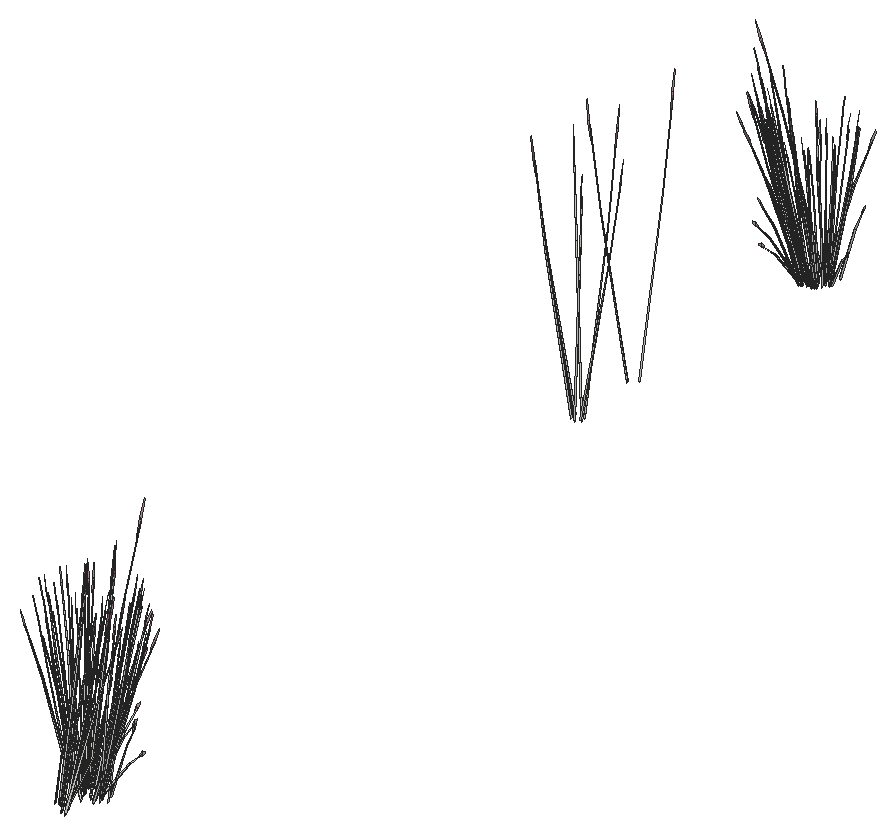
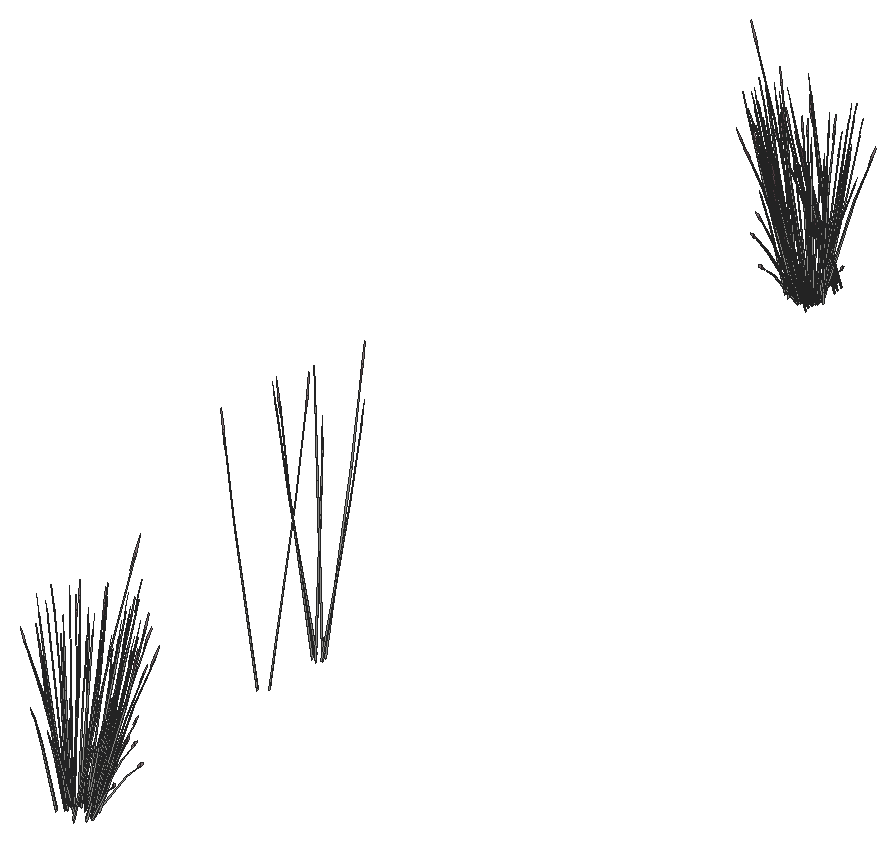
# SketchUp Ruby script. Lengths in inches.
U = 1.inch
M = Sketchup.active_model
def pt(a) = Geom::Point3d.new(a.map { |v| v * U })
def face(e, loops, mat)
  f = e.add_face(loops[0].map { |a| pt(a) })
  loops[1..].each { |l| e.add_face(l.map { |a| pt(a) }).erase! }
  f.material = f.back_material = mat if mat
  f
end
# faces: each face lists its corners as indices into pts; further lists are holes
def faces(e, pts, list, mat = nil) = list.each { |f| face(e, (f[0].is_a?(Array) ? f : [f]).map { |l| l.map { |i| pts[i] } }, mat) }
# xy, xz, yz: faces in a plane at the given z, y or x. An outline is a flat list of corners, or four numbers for a rectangle; further outlines are holes
def ring(l) = l.size == 4 ? [[l[0], l[1]], [l[2], l[1]], [l[2], l[3]], [l[0], l[3]]] : l.each_slice(2).to_a
def flat(e, list, mat, &to3) = list.each { |f| face(e, (f[0].is_a?(Array) ? f : [f]).map { |l| ring(l).map { |u, v| to3.(u, v) } }, mat) }
def xy(e, z, list, mat = nil) = flat(e, list, mat) { |x, y| [x, y, z] }
def xz(e, y, list, mat = nil) = flat(e, list, mat) { |x, z| [x, y, z] }
def yz(e, x, list, mat = nil) = flat(e, list, mat) { |y, z| [x, y, z] }
def lines(e, pts, list) = list.each { |a, b| e.add_line(pt(pts[a]), pt(pts[b])) }
# prism: a flat outline (further loops are holes) pulled along v
def prism(e, loops, v, mat = nil)
  f = face(e, loops, mat); d = Geom::Vector3d.new(v.map { |x| x * U })
  f.pushpull(f.normal.samedirection?(d) ? d.length : -d.length)
end
def box(e, o, s, mat = nil) = prism(e, [[o, [o[0] + s[0], o[1], o[2]], [o[0] + s[0], o[1] + s[1], o[2]], [o[0], o[1] + s[1], o[2]]]], [0, 0, s[2]], mat)
def at(x, y, z, deg = 0) = Geom::Transformation.translation(pt([x, y, z])) * Geom::Transformation.rotation(ORIGIN, Z_AXIS, deg.degrees)
def axes(o, x, y, z) = Geom::Transformation.new([*x, 0, *y, 0, *z, 0, *pt(o).to_a, 1])
def part(name) = M.definitions.add(name)
# library, detail: a bought-in or finely detailed component or shape, given as its bounding box
def library(name, o, s) = part(name).tap { |d| box(d.entities, o, s) }
def detail(e, o, s) = box(e.add_group.entities, o, s)
def put(e, d, t, mat = nil) = e.add_instance(d, t).tap { |i| i.material = mat if mat }
def group(e, t, mat = nil) = e.add_group.tap { |g| g.transformation = t; g.material = mat if mat }.entities
root = M.entities
M.materials.add("LightPink_Translucent").color = [144, 107, 117]
M.materials["LightPink_Translucent"].alpha = 0.75
c1 = part("blade")
p = [[2.15,0.21,22],[0,0.17,0],[0.09,0.45,0],[2.18,0.31,22],[2.29,0.31,22],[0.38,0.45,0],
  [2.48,0.24,33],[2.49,0.24,33],[2.48,0.22,33]]
faces(c1.entities,p,[[0,1,2,3],[4,5,2,3],[6,3,4,7],[8,0,3,6]])
c2 = part("seeds")
p = [[0.3,-0.1,1.38],[-0.01,-0.03,1.59],[-0.01,-0.03,0.03],[0.14,-0.07,-0.07],[0.29,-0.03,3],[0.15,0.01,3.11]]
faces(c2.entities,p,[[0,1,2,3],[1,0,4,5]],"LightPink_Translucent")
c3 = part("blade with seeds")
put(c3.entities,c1,at(0,0,0))
put(c3.entities,c2,axes([2.4,0.25,30.99],[1.5799,-0.05474,1.17369],[-0.12525,1.92788,0.29478],[-0.07173,-0.02425,1.56792]))
put(root,c3,axes([426.9,488.16,153.98],[-0.01019,0.09334,1.47793],[0.28908,0.3247,-0.23373],[-0.07568,0.15355,0.11853]))
put(root,c3,axes([427.82,487.95,154.56],[0.45039,0.02337,-0.11403],[-0.01231,0.44247,-0.63292],[-0.03129,0.17041,0.9617]))
put(root,c3,axes([428.66,488.45,154.25],[0.40102,-0.2196,-0.10273],[0.19707,0.38974,-0.57019],[0.05291,0.16424,0.8664]))
put(root,c3,axes([427.625,491.67,153.95],[-0.29757,0.31243,-0.43168],[-0.2606,-0.33005,-0.33437],[-0.15119,-0.04754,0.82598]))
put(root,c3,axes([427.78,491.35,154.25],[-0.02194,0.47967,-0.10273],[-0.41546,-0.01311,-0.57019],[-0.16001,-0.03332,0.8664]))
put(root,c3,axes([430.89,493.1875,154.25],[-0.20619,-0.42709,-0.10273],[0.36595,-0.20988,-0.57019],[0.15422,-0.05635,0.8664]))
put(root,c3,axes([430.87,492.82,153.95],[0.11102,-0.42903,-0.43168],[0.38064,0.14706,-0.33437],[0.15325,-0.03934,0.82598]))
put(root,c3,axes([428.13,488.12,154.23],[0.29336,0.31691,-0.47917],[-0.3099,0.27755,-0.37115],[-0.04464,0.16102,0.91684]))
put(root,c3,axes([427.25,492.01,153.27],[0.16998,-0.01068,1.44779],[-0.11276,0.46299,0.11706],[-0.24224,-0.02864,0.61892]))
put(root,c3,axes([429,488.43,153.95],[0.40284,0.11824,-0.43168],[-0.13808,0.40538,-0.33437],[0.03694,0.16321,0.82598]))
put(root,c3,axes([429.23,487.59,153.27],[-0.09368,-0.15143,1.44779],[0.43286,-0.12749,0.11706],[0.09783,0.23774,0.61892]))
put(root,c3,axes([428.82,488.68,153.82],[-0.12355,0.36271,-0.29918],[-0.36044,-0.10579,0.38624],[0.03305,0.14603,0.73904]))
put(root,c3,axes([430.8,492.98,154.21],[0.3601,-0.20831,-0.60019],[0.20068,0.4288,0.07243],[0.17399,-0.04871,0.84903]))
put(root,c3,axes([428.04,487.97,154.51],[-0.01066,0.43628,-0.66621],[-0.44902,-0.0293,0.0804],[-0.04739,0.18483,0.94242]))
put(root,c3,axes([426.87,489.12,153.98],[0.04649,-0.02848,1.49853],[0.38427,0.18941,-0.1416],[-0.00903,0.15771,0.26519]))
put(root,c3,axes([428.46,487.67,153.27],[-0.01003,-0.18103,1.44779],[0.43473,0.12009,0.11706],[-0.02689,0.25798,0.61892]))
put(root,c3,axes([427.18,492.36,154],[0.11578,-0.43006,0.40553],[0.38064,0.14706,0.33437],[-0.14969,0.02584,0.83914]))
put(root,c3,axes([428.85,488.35,154.21],[0.19559,0.38351,-0.60019],[-0.40262,0.21373,0.07243],[0.04574,0.1853,0.84903]))
put(root,c3,axes([427.15,492.24,154],[-0.15051,-0.3216,0.05432],[0.27447,-0.15741,0.42765],[-0.12099,0.03106,0.65209]))
put(root,c3,axes([428.5625,489.32,153.98],[0.05195,0.07595,1.47793],[0.41921,0.02984,-0.23373],[0.04216,0.1675,0.11853]))
put(root,c3,axes([431.1,493.02,153.82],[0.34057,0.13158,-0.29918],[-0.09933,0.38387,0.38624],[0.13712,-0.0352,0.73904]))
put(root,c3,axes([427.1,492.4,153.82],[-0.34057,-0.13158,-0.29918],[0.09933,-0.38387,0.38624],[-0.13712,0.0352,0.73904]))
put(root,c3,axes([427.89,488.59,152.84],[0.009,-0.24349,1.30391],[0.40497,0.12861,0.18019],[-0.03509,0.2595,0.61571]))
put(root,c3,axes([430.18,492.54,153.27],[-0.16998,0.01068,1.44779],[0.11276,-0.46299,0.11706],[0.24224,0.02864,0.61892]))
put(root,c3,axes([431.05,493.18,154],[0.15051,0.3216,0.05432],[-0.27447,0.15741,0.42765],[0.12099,-0.03106,0.65209]))
put(root,c3,axes([431.03,493.0625,154],[-0.11578,0.43006,0.40553],[-0.38064,-0.14706,0.33437],[0.14969,-0.02584,0.83914]))
put(root,c3,axes([428.14,492.34,152.82],[0.11649,-0.06823,1.49584],[0.04017,0.47639,0.11706],[-0.25231,0.06321,0.53462]))
put(root,c3,axes([431.71,494.46,153.98],[-0.03706,-0.04129,1.49853],[0.08106,-0.44261,-0.1416],[0.14596,-0.02828,0.26519]))
put(root,c3,axes([426.89,492.66,153.98],[-0.06692,0.06124,1.47793],[0.00569,0.44742,-0.23373],[-0.15339,0.05818,0.11853]))
put(root,c3,axes([427.34,492.6,153.95],[-0.11102,0.42903,-0.43168],[-0.38064,-0.14706,-0.33437],[-0.15325,0.03934,0.82598]))
put(root,c3,axes([427.32,492.23,154.25],[0.20619,0.42709,-0.10273],[-0.36595,0.20988,-0.57019],[-0.15422,0.05635,0.8664]))
put(root,c3,axes([431.39,494.09,153.32],[-0.07843,-0.39649,-0.0295],[0.37072,-0.09115,-0.13375],[0.07742,0.02514,0.44114]))
put(root,c3,axes([430.43,494.07,154.25],[0.02194,-0.47967,-0.10273],[0.41546,0.01311,-0.57019],[0.16001,0.03332,0.8664]))
put(root,c3,axes([430.79,493.79,153.98],[0.08791,-0.00798,1.47793],[0.24113,-0.36643,-0.23373],[0.15637,0.04837,0.11853]))
put(root,c3,axes([427.27,493.43,154],[-0.10163,-0.43409,0.40553],[0.39868,-0.07534,0.33437],[-0.1175,0.10209,0.83914]))
put(root,c3,axes([427.19,493.34,154],[-0.28133,-0.19836,0.05432],[0.16379,-0.28248,0.42765],[-0.0902,0.09132,0.65209]))
put(root,c3,axes([427.32,492.82,153.27],[0.14219,-0.09977,1.44779],[0.11971,0.461,0.11706],[-0.22323,0.10419,0.61892]))
put(root,c3,axes([430.45,493.84,154.21],[0.40965,0.01136,-0.60019],[-0.02751,0.47821,0.07243],[0.17355,0.05047,0.84903]))
put(root,c3,axes([426.14,493.11,153.98],[0.0523,0.01265,1.49853],[0.16179,0.41674,-0.1416],[-0.10706,0.10938,0.26519]))
put(root,c3,axes([430.69,494.04,153.82],[0.23317,0.29531,-0.29918],[-0.26625,0.27955,0.38624],[0.13527,0.04253,0.73904]))
put(root,c3,axes([430.57,494.15,154],[-0.02064,0.35866,0.05432],[-0.3116,-0.00983,0.42765],[0.11936,0.03753,0.65209]))
put(root,c3,axes([427.23,493.51,153.82],[-0.35672,0.06741,-0.29918],[-0.09419,-0.38534,0.38624],[-0.10222,0.1035,0.73904]))
put(root,c3,axes([430.6,494.04,154],[-0.30217,0.31079,0.40553],[-0.2606,-0.33005,0.33437],[0.14177,0.05733,0.83914]))
put(root,c3,axes([429.86,493.28,153.27],[-0.15222,-0.08126,1.44779],[0.31502,-0.34091,0.11706],[0.19634,0.15379,0.61892]))
put(root,c3,axes([429.88,492.21,153.78],[-0.35411,-0.24507,1.16821],[0.37391,-0.38156,0.50405],[0.11425,0.22994,1.12919]))
put(root,c3,axes([427.33,493.25,154.25],[0.37908,0.26007,-0.10273],[-0.21839,0.37663,-0.57019],[-0.1071,0.13092,0.8664]))
put(root,c3,axes([429.61,494.6,154.25],[0.2442,-0.40372,-0.10273],[0.35364,0.23259,-0.57019],[0.12293,0.11406,0.8664]))
put(root,c3,axes([427.84,493.13,153.27],[0.10236,-0.14492,1.44779],[0.25844,0.39118,0.11706],[-0.17726,0.17814,0.61892]))
put(root,c3,axes([427.52,493.56,153.95],[0.10528,0.43067,-0.43168],[-0.39868,0.07534,-0.33437],[-0.11425,0.11568,0.82598]))
put(root,c3,axes([429.29,494.93,153.98],[0.00121,-0.0571,1.49853],[0.35119,-0.25193,-0.1416],[0.12199,0.08992,0.26519]))
put(root,c3,axes([427.75,494.28,154],[-0.33677,-0.02198,0.05432],[0.00923,-0.33185,0.42765],[-0.03524,0.12712,0.65209]))
put(root,c3,axes([427.85,494.31,154],[-0.29182,-0.32181,0.40553],[0.3099,-0.27755,0.33437],[-0.05383,0.15098,0.83914]))
put(root,c3,axes([429.9,494.4,153.95],[0.40438,-0.11212,-0.43168],[0.07074,0.4246,-0.33437],[0.10862,0.12168,0.82598]))
put(root,c3,axes([429.7,494.74,154],[-0.18625,0.29962,0.05432],[-0.26523,-0.17444,0.42765],[0.08575,0.09606,0.65209]))
put(root,c3,axes([429.78,494.66,154],[-0.4076,0.10824,0.40553],[-0.07074,-0.4246,0.33437],[0.09586,0.12514,0.83914]))
put(root,c3,axes([427.77,493.49,153.27],[0.0763,-0.16212,1.44779],[0.3201,0.3355,0.11706],[-0.1444,0.2091,0.61892]))
put(root,c3,axes([428.66,494.79,154],[-0.30197,0.1603,0.05432],[-0.1478,-0.29231,0.42765],[0.02916,0.12885,0.65209]))
put(root,c3,axes([427.85,494.4,153.82],[-0.27728,0.24833,-0.29918],[-0.26248,-0.28355,0.38624],[-0.03994,0.14407,0.73904]))
put(root,c3,axes([426.9,494.33,153.98],[-0.01019,0.09334,1.47793],[0.28908,0.3247,-0.23373],[-0.07568,0.15355,0.11853]))
put(root,c3,axes([427.82,494.12,154.56],[0.45039,0.02337,-0.11403],[-0.01231,0.44247,-0.63292],[-0.03129,0.17041,0.9617]))
put(root,c3,axes([428.66,494.61,154.25],[0.40102,-0.2196,-0.10273],[0.19707,0.38974,-0.57019],[0.05291,0.16424,0.8664]))
put(root,c3,axes([428.13,494.29,154.23],[0.29336,0.31691,-0.47917],[-0.3099,0.27755,-0.37115],[-0.04464,0.16102,0.91684]))
put(root,c3,axes([429,494.59,153.95],[0.40284,0.11824,-0.43168],[-0.13808,0.40538,-0.33437],[0.03694,0.16321,0.82598]))
put(root,c3,axes([429.23,493.76,153.27],[-0.09368,-0.15143,1.44779],[0.43286,-0.12749,0.11706],[0.09783,0.23774,0.61892]))
put(root,c3,axes([428.82,494.84,153.82],[-0.12355,0.36271,-0.29918],[-0.36044,-0.10579,0.38624],[0.03305,0.14603,0.73904]))
put(root,c3,axes([428.04,494.14,154.51],[-0.01066,0.43628,-0.66621],[-0.44902,-0.0293,0.0804],[-0.04739,0.18483,0.94242]))
put(root,c3,axes([426.87,495.29,153.98],[0.04649,-0.02848,1.49853],[0.38427,0.18941,-0.1416],[-0.00903,0.15771,0.26519]))
put(root,c3,axes([428.46,493.83,153.27],[-0.01003,-0.18103,1.44779],[0.43473,0.12009,0.11706],[-0.02689,0.25798,0.61892]))
put(root,c3,axes([428.85,494.52,154.21],[0.19559,0.38351,-0.60019],[-0.40262,0.21373,0.07243],[0.04574,0.1853,0.84903]))
put(root,c3,axes([428.5625,495.48,153.98],[0.05195,0.07595,1.47793],[0.41921,0.02984,-0.23373],[0.04216,0.1675,0.11853]))
put(root,c3,axes([427.89,494.76,152.84],[0.009,-0.24349,1.30391],[0.40497,0.12861,0.18019],[-0.03509,0.2595,0.61571]))
put(root,c3,axes([416.45,611.06,155.27],[-0.1683,-0.48366,-0.58997],[0.48479,-0.17419,-0.15484],[-0.0186,-0.16378,1.30225]))
put(root,c3,axes([417.19,610.5625,155.23],[0.27603,-0.35451,-0.52676],[0.34289,0.32147,-0.13825],[0.11061,-0.08844,1.16273]))
put(root,c3,axes([416.51,611.96,155.23],[-0.42629,-0.07733,-0.52676],[0.08996,-0.47699,-0.13825],[-0.12722,-0.0578,1.16273]))
put(root,c3,axes([417.94,610.97,155.23],[0.42629,0.07733,-0.52676],[-0.08996,0.47699,-0.13825],[0.12722,0.0578,1.16273]))
put(root,c3,axes([417.27,612.375,155.23],[-0.27603,0.35451,-0.52676],[-0.34289,-0.32147,-0.13825],[-0.11061,0.08844,1.16273]))
put(root,c3,axes([417.99,611.88,155.26],[0.15027,0.43184,-0.5847],[-0.43285,0.15553,-0.15346],[0.01661,0.14623,1.29063]))
put(root,c3,axes([416.45,622.8125,155.625],[-0.1683,-0.48366,-0.58997],[0.48479,-0.17419,-0.15484],[-0.0186,-0.16378,1.30225]))
put(root,c3,axes([417.99,623.63,155.62],[0.15027,0.43184,-0.5847],[-0.43285,0.15553,-0.15346],[0.01661,0.14623,1.29063]))
put(root,c3,axes([416.2,660.48,153.27],[0.09368,0.15143,1.44779],[-0.43286,0.12749,0.11706],[-0.09783,-0.23774,0.61892]))
put(root,c3,axes([416.91,659.47,153.98],[-0.06268,-0.06613,1.47793],[-0.4183,0.04193,-0.23373],[-0.06676,-0.15817,0.11853]))
put(root,c3,axes([417.35,660.59,154.21],[-0.19559,-0.38351,-0.60019],[0.40262,-0.21373,0.07243],[-0.04574,-0.1853,0.84903]))
put(root,c3,axes([418.17,660.96,154.21],[0.01066,-0.43628,-0.60019],[0.44902,0.0293,0.07243],[0.04739,-0.18483,0.84903]))
put(root,c3,axes([418.79,660.28,153.98],[-0.00396,-0.09387,1.47793],[-0.33411,-0.2713,-0.23373],[0.05166,-0.16446,0.11853]))
put(root,c3,axes([417.39,660.26,153.82],[0.12355,-0.36271,-0.29918],[0.36044,0.10579,0.38624],[-0.03305,-0.14603,0.73904]))
put(root,c3,axes([417.66,660.74,153.27],[-0.0763,0.16212,1.44779],[-0.3201,-0.3355,0.11706],[0.1444,-0.2091,0.61892]))
put(root,c3,axes([418.7,659.95,153.98],[-0.04162,0.03603,1.49853],[-0.40776,-0.12155,-0.1416],[-0.01476,-0.15722,0.26519]))
put(root,c3,axes([417.21,660.51,153.95],[-0.40284,-0.11824,-0.43168],[0.13808,-0.40538,-0.33437],[-0.03694,-0.16321,0.82598]))
put(root,c3,axes([418.08,660.82,153.95],[-0.29336,-0.31691,-0.43168],[0.3099,-0.27755,-0.33437],[0.04464,-0.16102,0.82598]))
put(root,c3,axes([416.49,659.25,153.98],[-0.00765,0.05653,1.49853],[-0.37706,0.20517,-0.1416],[-0.11096,-0.10488,0.26519]))
put(root,c3,axes([417.55,660.49,154.25],[-0.40102,0.2196,-0.10273],[-0.19707,-0.38974,-0.57019],[-0.05291,-0.16424,0.8664]))
put(root,c3,axes([418.38,660.99,154.25],[-0.45039,-0.02337,-0.10273],[0.01231,-0.44247,-0.57019],[0.03129,-0.17041,0.8664]))
put(root,c3,axes([418.35,660.7,153.82],[0.27728,-0.24833,-0.29918],[0.26248,0.28355,0.38624],[0.03994,-0.14407,0.73904]))
put(root,c3,axes([417.54,660.32,154],[0.30197,-0.1603,0.05432],[0.1478,0.29231,0.42765],[-0.02916,-0.12885,0.65209]))
put(root,c3,axes([416.47,660.7,154.21],[-0.34944,-0.22798,-0.60019],[0.24834,-0.39949,0.07243],[-0.1266,-0.13612,0.84903]))
put(root,c3,axes([416.35,660.4,153.82],[-0.06329,-0.37991,-0.29918],[0.36182,-0.10032,0.38624],[-0.09718,-0.10887,0.73904]))
put(root,c3,axes([416.51,660.36,154],[0.18625,-0.29962,0.05432],[0.26523,0.17444,0.42765],[-0.08575,-0.09606,0.65209]))
put(root,c3,axes([415.57,660.95,153.27],[0.15222,0.08126,1.44779],[-0.31502,0.34091,0.11706],[-0.19634,-0.15379,0.61892]))
put(root,c3,axes([416.31,660.71,153.95],[-0.40438,0.11212,-0.43168],[-0.07074,-0.4246,-0.33437],[-0.10862,-0.12168,0.82598]))
put(root,c3,axes([416.59,660.33,154.59],[-0.2735,0.45217,-0.11506],[-0.39608,-0.2605,-0.63862],[-0.13768,-0.12775,0.97037]))
put(root,c3,axes([418.46,660.83,154],[0.33677,0.02198,0.05432],[-0.00923,0.33185,0.42765],[0.03524,-0.12712,0.65209]))
put(root,c3,axes([418.7,661.72,154.21],[0.21406,-0.37215,-0.60019],[0.37511,0.26448,0.07243],[0.12781,-0.13483,0.84903]))
put(root,c3,axes([418.6875,661.55,153.95],[-0.10528,-0.43067,-0.43168],[0.39868,-0.07534,-0.33437],[0.11425,-0.11568,0.82598]))
put(root,c3,axes([415.54,660.2,153.98],[-0.08817,-0.00333,1.47793],[-0.28072,0.33293,-0.23373],[-0.14978,-0.06803,0.11853]))
put(root,c3,axes([418.875,661.86,154.25],[-0.37908,-0.26007,-0.10273],[0.21839,-0.37663,-0.57019],[0.1071,-0.13092,0.8664]))
put(root,c3,axes([417.31,663.28,152.81],[0.35414,0.19019,1.27785],[-0.34693,0.40974,0.50532],[-0.1554,-0.24285,1.07126]))
put(root,c3,axes([419.81,661.74,153.98],[-0.05353,-0.00358,1.49853],[-0.22227,-0.38383,-0.1416],[0.08926,-0.1262,0.26519]))
put(root,c3,axes([418.98,661.59,153.82],[0.35672,-0.06741,-0.29918],[0.09419,0.38534,0.38624],[0.10222,-0.1035,0.73904]))
put(root,c3,axes([415.63,660.95,154],[0.02064,-0.35866,0.05432],[0.3116,0.00983,0.42765],[-0.11936,-0.03753,0.65209]))
put(root,c3,axes([415.51,661.0625,153.82],[-0.23317,-0.29531,-0.29918],[0.26625,-0.27955,0.38624],[-0.13527,-0.04253,0.73904]))
put(root,c3,axes([415.76,661.26,154.21],[-0.40965,-0.01136,-0.60019],[0.02751,-0.47821,0.07243],[-0.17355,-0.05047,0.84903]))
put(root,c3,axes([419.01,661.76,154],[0.28133,0.19836,0.05432],[-0.16379,0.28248,0.42765],[0.0902,-0.09132,0.65209]))
put(root,c3,axes([420.01,662.2,153.98],[0.05687,-0.07184,1.47793],[-0.07279,-0.44069,-0.23373],[0.14268,-0.08356,0.11853]))
put(root,c3,axes([415.2,660.48,153.98],[0.03038,0.04707,1.49853],[-0.14646,0.42312,-0.1416],[-0.14833,0.00306,0.26519]))
put(root,c3,axes([415.625,661.36,153.95],[-0.29757,0.31243,-0.43168],[-0.2606,-0.33005,-0.33437],[-0.15119,-0.04754,0.82598]))
put(root,c3,axes([415.78,661.03,154.25],[-0.02194,0.47967,-0.10273],[-0.41546,-0.01311,-0.57019],[-0.16001,-0.03332,0.8664]))
put(root,c3,axes([418.89,662.87,154.25],[-0.20619,-0.42709,-0.10273],[0.36595,-0.20988,-0.57019],[0.15422,-0.05635,0.8664]))
put(root,c3,axes([418.87,662.5,153.95],[0.11102,-0.42903,-0.43168],[0.38064,0.14706,-0.33437],[0.15325,-0.03934,0.82598]))
put(root,c3,axes([415.25,661.69,153.27],[0.16998,-0.01068,1.44779],[-0.11276,0.46299,0.11706],[-0.24224,-0.02864,0.61892]))
put(root,c3,axes([418.8,662.66,154.21],[0.3601,-0.20831,-0.60019],[0.20068,0.4288,0.07243],[0.17399,-0.04871,0.84903]))
put(root,c3,axes([415.15,661.93,154],[-0.15051,-0.3216,0.05432],[0.27447,-0.15741,0.42765],[-0.12099,0.03106,0.65209]))
put(root,c3,axes([419.1,662.7,153.82],[0.34057,0.13158,-0.29918],[-0.09933,0.38387,0.38624],[0.13712,-0.0352,0.73904]))
put(root,c3,axes([415.1,662.09,153.82],[-0.34057,-0.13158,-0.29918],[0.09933,-0.38387,0.38624],[-0.13712,0.0352,0.73904]))
put(root,c3,axes([418.18,662.23,153.27],[-0.16998,0.01068,1.44779],[0.11276,-0.46299,0.11706],[0.24224,0.02864,0.61892]))
put(root,c3,axes([419.05,662.86,154],[0.15051,0.3216,0.05432],[-0.27447,0.15741,0.42765],[0.12099,-0.03106,0.65209]))
put(root,c3,axes([416.14,662.02,152.82],[0.11649,-0.06823,1.49584],[0.04017,0.47639,0.11706],[-0.25231,0.06321,0.53462]))
put(root,c3,axes([419.71,664.14,153.98],[-0.03706,-0.04129,1.49853],[0.08106,-0.44261,-0.1416],[0.14596,-0.02828,0.26519]))
put(root,c3,axes([414.89,662.34,153.98],[-0.06692,0.06124,1.47793],[0.00569,0.44742,-0.23373],[-0.15339,0.05818,0.11853]))
put(root,c3,axes([415.34,662.28,153.95],[-0.11102,0.42903,-0.43168],[-0.38064,-0.14706,-0.33437],[-0.15325,0.03934,0.82598]))
